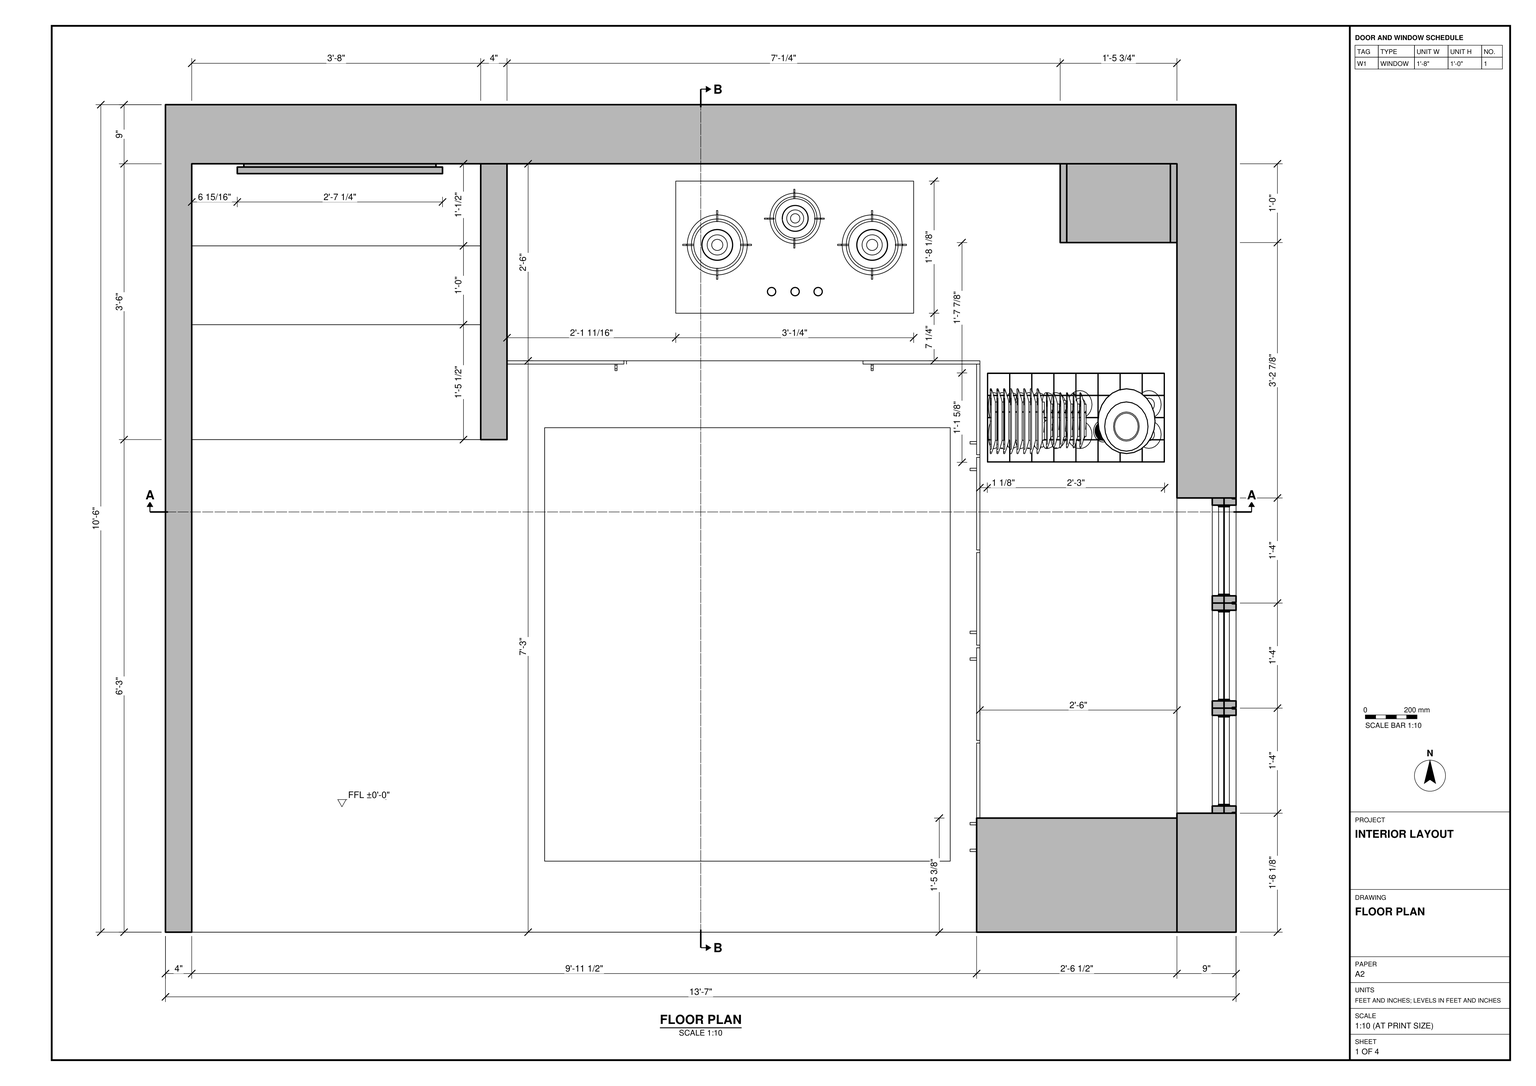
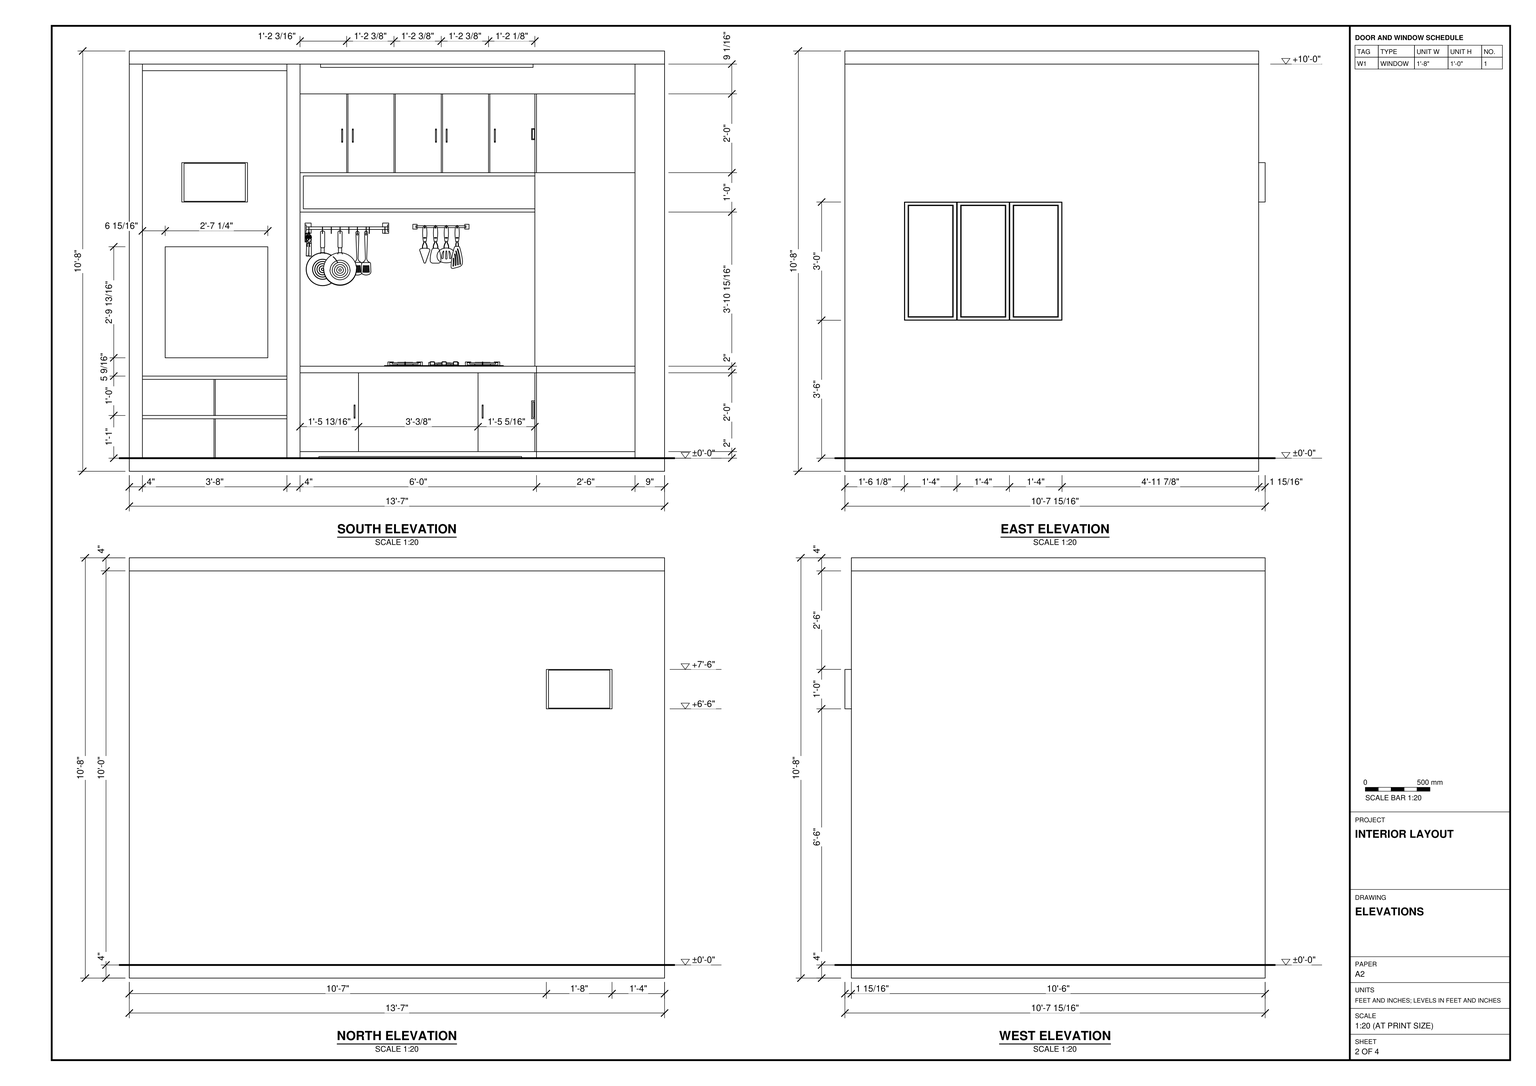
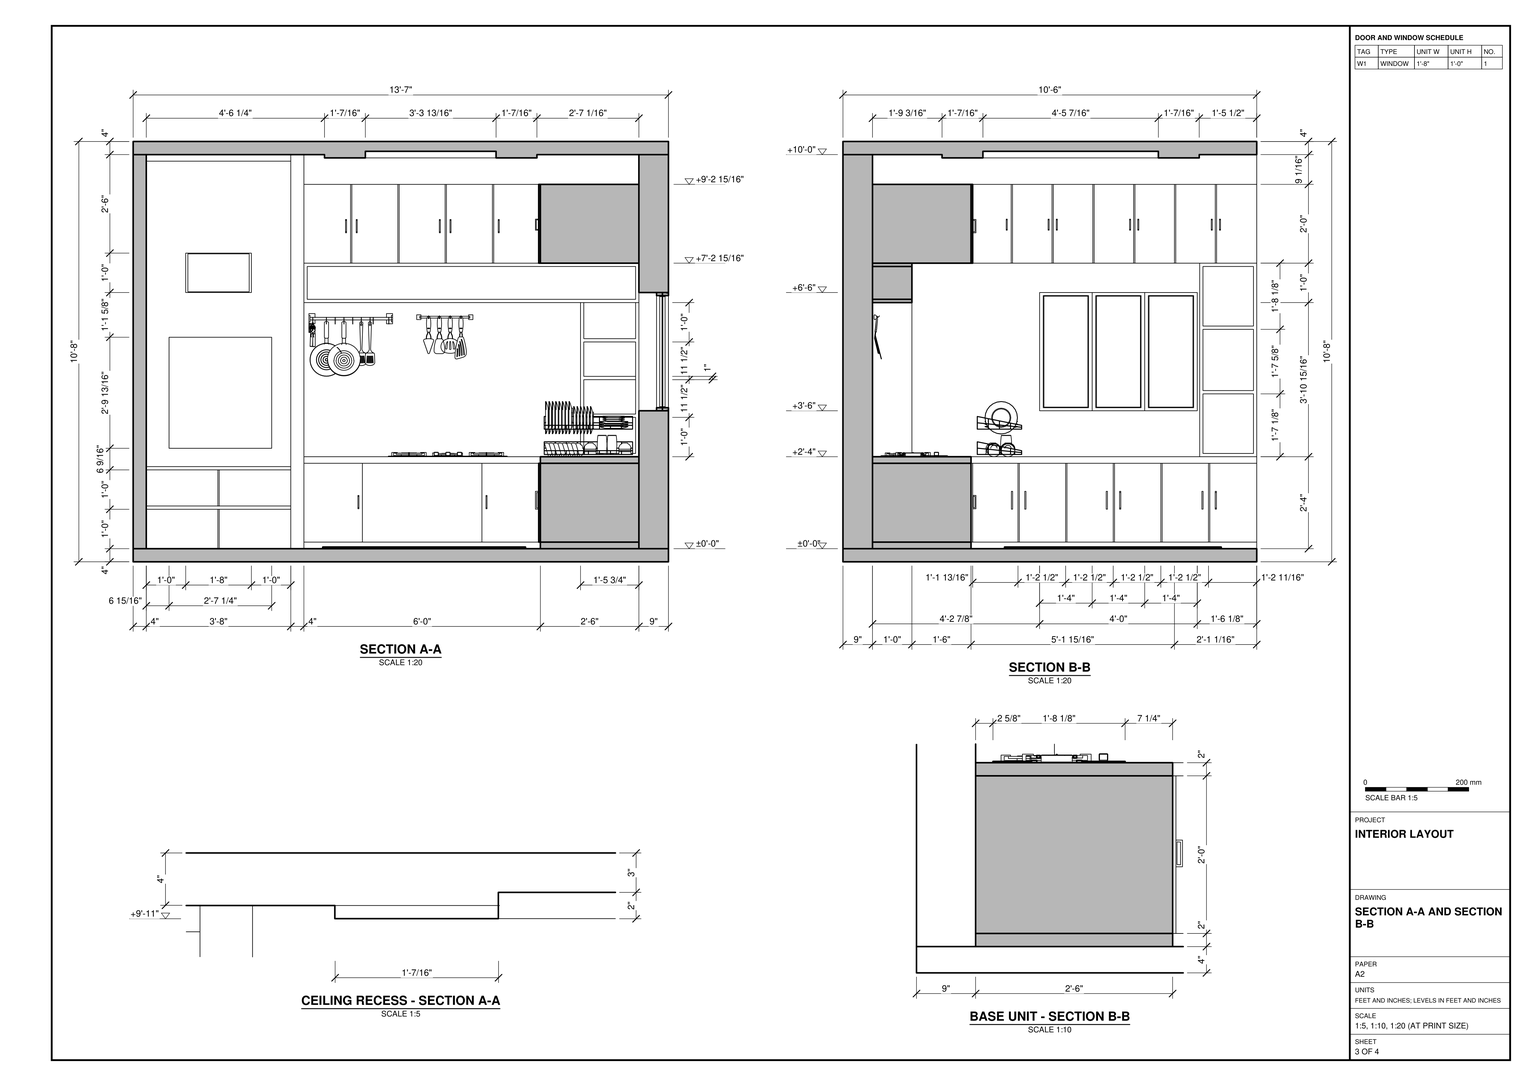
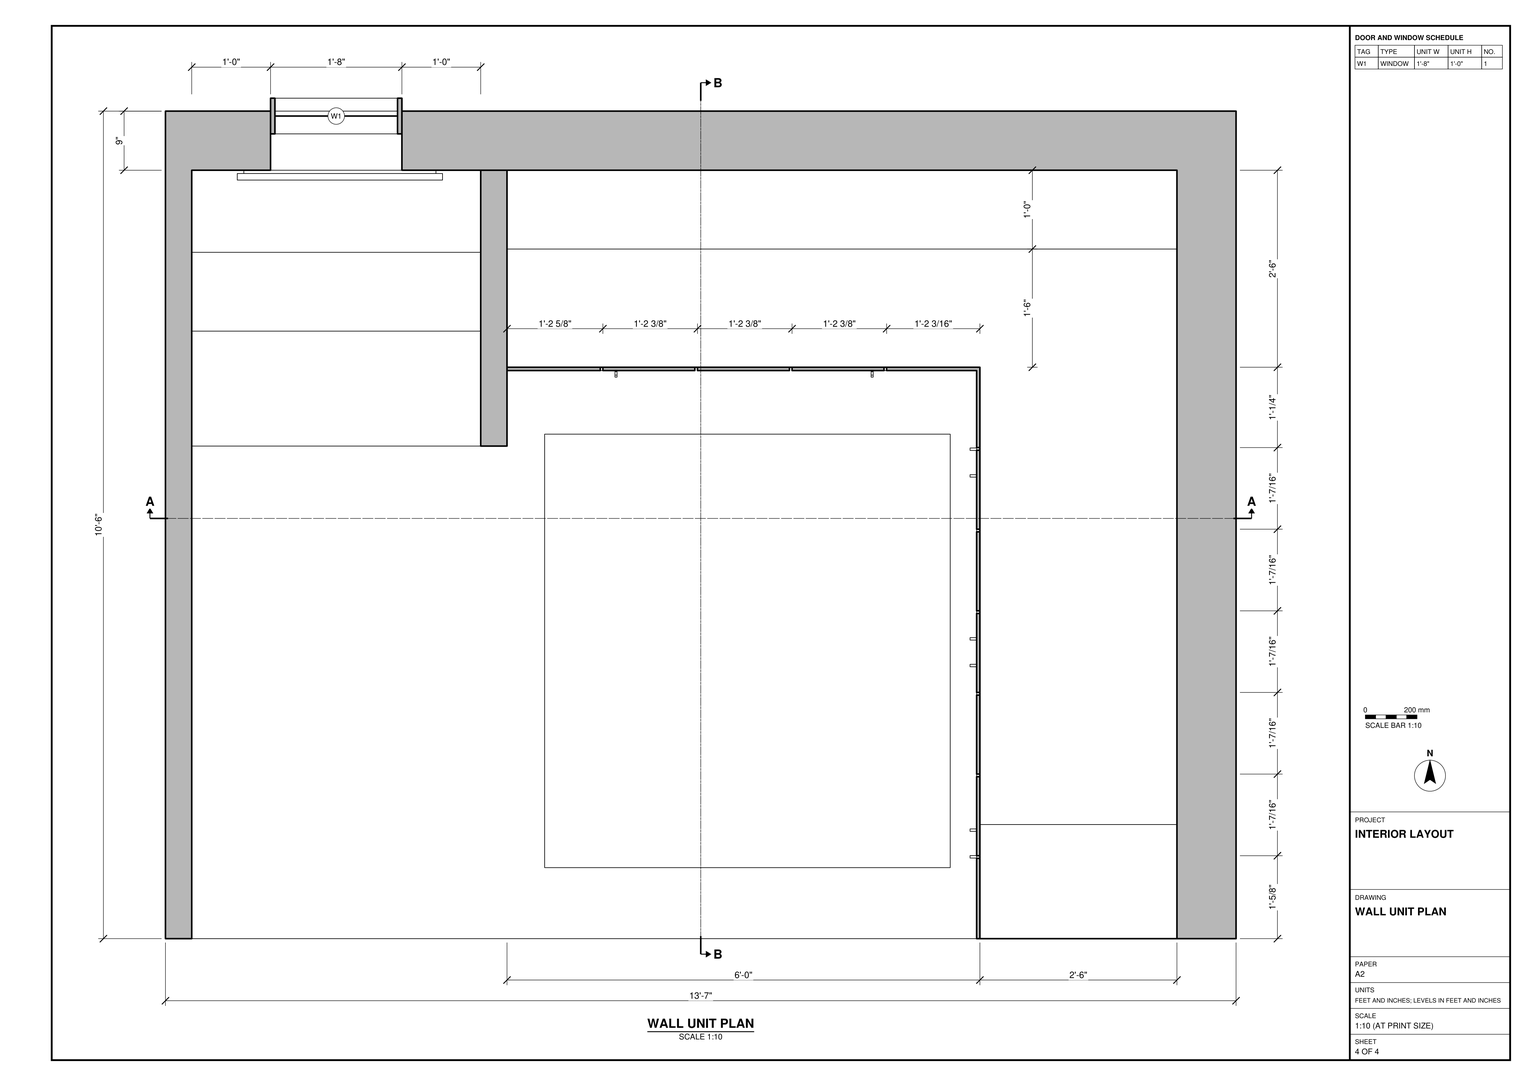
Build the kitchen interior in SketchUp from task_files/diagram_01.pdf. Work in feet and inches. The overall model extents are 13'-7" east to west, 10'-7 15/16" north to south and 10'-8" high. Set the single finished floor level at ±0'-0".

Use the floor plan for the wall positions and the sections for the floor slab, ceiling slab and ceiling recesses. Keep the south side open as drawn. Use 9" walls on the north and east, and 4" walls for the west side and the short partition beside the storage alcove. Model the small high window in the alcove and the three-panel glazed opening above the east counter.

Fit the base cabinets and continuous worktop along the north and east walls, leaving the centre of the room clear. Use the sections to set the counter height, cabinet fronts, plinths, pulls, upper cupboards and open shelves. Include the low divided shelving and wall panel in the alcove. Place the cooktop on the north counter, the hanging utensils above it and the dish rack near the corner on the east return. Decor and loose items may be any suitable library components, for example from 3D Warehouse.

Keep the shell elements and each joinery or furniture piece in separate groups or components, and use components for repeated parts. Save one SketchUp model as output_files/kitchen_with_l_shaped_cabinetry_and_storage_alcove.skp.

# SketchUp Ruby script. Lengths in inches.
U = 1.inch
M = Sketchup.active_model
def pt(a) = Geom::Point3d.new(a.map { |v| v * U })
def face(e, loops, mat)
  f = e.add_face(loops[0].map { |a| pt(a) })
  loops[1..].each { |l| e.add_face(l.map { |a| pt(a) }).erase! }
  f.material = f.back_material = mat if mat
  f
end
# faces: each face lists its corners as indices into pts; further lists are holes
def faces(e, pts, list, mat = nil) = list.each { |f| face(e, (f[0].is_a?(Array) ? f : [f]).map { |l| l.map { |i| pts[i] } }, mat) }
# xy, xz, yz: faces in a plane at the given z, y or x. An outline is a flat list of corners, or four numbers for a rectangle; further outlines are holes
def ring(l) = l.size == 4 ? [[l[0], l[1]], [l[2], l[1]], [l[2], l[3]], [l[0], l[3]]] : l.each_slice(2).to_a
def flat(e, list, mat, &to3) = list.each { |f| face(e, (f[0].is_a?(Array) ? f : [f]).map { |l| ring(l).map { |u, v| to3.(u, v) } }, mat) }
def xy(e, z, list, mat = nil) = flat(e, list, mat) { |x, y| [x, y, z] }
def xz(e, y, list, mat = nil) = flat(e, list, mat) { |x, z| [x, y, z] }
def yz(e, x, list, mat = nil) = flat(e, list, mat) { |y, z| [x, y, z] }
def lines(e, pts, list) = list.each { |a, b| e.add_line(pt(pts[a]), pt(pts[b])) }
# prism: a flat outline (further loops are holes) pulled along v
def prism(e, loops, v, mat = nil)
  f = face(e, loops, mat); d = Geom::Vector3d.new(v.map { |x| x * U })
  f.pushpull(f.normal.samedirection?(d) ? d.length : -d.length)
end
def box(e, o, s, mat = nil) = prism(e, [[o, [o[0] + s[0], o[1], o[2]], [o[0] + s[0], o[1] + s[1], o[2]], [o[0], o[1] + s[1], o[2]]]], [0, 0, s[2]], mat)
def at(x, y, z, deg = 0) = Geom::Transformation.translation(pt([x, y, z])) * Geom::Transformation.rotation(ORIGIN, Z_AXIS, deg.degrees)
def axes(o, x, y, z) = Geom::Transformation.new([*x, 0, *y, 0, *z, 0, *pt(o).to_a, 1])
def part(name) = M.definitions.add(name)
# library, detail: a bought-in or finely detailed component or shape, given as its bounding box
def library(name, o, s) = part(name).tap { |d| box(d.entities, o, s) }
def detail(e, o, s) = box(e.add_group.entities, o, s)
def put(e, d, t, mat = nil) = e.add_instance(d, t).tap { |i| i.material = mat if mat }
def group(e, t, mat = nil) = e.add_group.tap { |g| g.transformation = t; g.material = mat if mat }.entities
root = M.entities
M.materials.add("Emissive").color = [214, 204, 90]
M.materials.add("Wine2").color = [0, 0, 0]
M.materials["Wine2"].alpha = 0
M.materials.add("[0048_PaleGoldenrod]").color = [238, 232, 170]
M.materials.add("[0052_FloralWhite]").color = [255, 250, 240]
M.materials.add("[0055_LightGoldenrodYellow]").color = [250, 250, 210]
M.materials.add("[0057_DarkKhaki]").color = [189, 183, 107]
M.materials.add("[0130_Gainsboro]").color = [39, 45, 50]
M.materials.add("[Aluminum]").color = [179, 179, 179]
M.materials.add("[Carrera Marble]").color = [207, 207, 207]
M.materials.add("[Color M07]").color = [58, 58, 58]
M.materials.add("[Granite Dark Gray]").color = [69, 68, 68]
M.materials.add("[Stone Brushed Khaki]").color = [226, 197, 133]
M.materials.add("[Stone Vein Gray]").color = [166, 165, 165]
M.materials.add("[Textile Leaves Green]").color = [158, 160, 98]
M.materials.add("[Translucent Glass Gray]3").color = [128, 128, 128]
M.materials["[Translucent Glass Gray]3"].alpha = 0.3
M.materials.add("[Translucent Glass Sky Reflection]").color = [126, 138, 183]
M.materials["[Translucent Glass Sky Reflection]"].alpha = 0.52
c1 = part("Group14\#1")
p = [[0,0,0],[0,0,-15.5],[-7.68,0,-15.5],[50,-0.18,0],[-50,-0.18,0],[50,0.18,0],
  [50,0,0],[-50,0.18,0],[7.68,0,-15.5],[-50,0,0],[0,0,-25.09]]
lines(c1.entities,p,[[0,1],[1,2],[3,4],[5,6],[7,5],[1,8],[9,0],[0,6],[8,10],[4,9],[6,3],[2,10],
  [9,7]])
c2 = part("Rectangle Light")
put(c2.entities,c1,at(0,0,0))
c3 = part("WINDOW (1)")
xy(c3.entities,0,[[0,0,59.06,1.97]],"[Color M07]")
xy(c3.entities,1.97,[[1.97,0,57.09,0.98],[1.97,0.98,57.09,1.97]],"[Color M07]")
xy(c3.entities,104.33,[[1.97,0,57.09,0.98],[1.97,0.98,57.09,1.97]],"[Color M07]")
xy(c3.entities,106.3,[[0,0,59.06,1.97]],"[Color M07]")
xz(c3.entities,0,[[[0,0,59.06,106.3],[1.97,1.97,57.09,104.33]]],"[Color M07]")
xz(c3.entities,0.98,[[1.97,1.97,57.09,104.33]],"[Translucent Glass Gray]3")
xz(c3.entities,1.97,[[[0,0,59.06,106.3],[1.97,1.97,57.09,104.33]]],"[Color M07]")
yz(c3.entities,0,[[0,0,1.97,106.3]],"[Color M07]")
yz(c3.entities,1.97,[[0,1.97,0.98,104.33],[0.98,1.97,1.97,104.33]],"[Color M07]")
yz(c3.entities,57.09,[[0,1.97,0.98,104.33],[0.98,1.97,1.97,104.33]],"[Color M07]")
yz(c3.entities,59.06,[[0,0,1.97,106.3]],"[Color M07]")
c4 = part("Framed panel")
xy(c4.entities,0,[[0,-0.98,43.07,0],[0,0,43.07,1.4]],"[0130_Gainsboro]")
xy(c4.entities,0.3,[[0.3,-1.43,42.77,-0.98]],"[0130_Gainsboro]")
xy(c4.entities,2.95,[[2.95,-1.43,40.12,-0.63],[2.95,-0.63,40.12,0],[2.95,0,40.12,0.64],[2.95,0.64,40.12,1.4]],"[0130_Gainsboro]")
xy(c4.entities,3.54,[[3.54,-0.63,39.53,0],[3.54,0,39.53,0.64]],"[0130_Gainsboro]")
xy(c4.entities,111.8125,[[3.54,-0.63,39.53,0],[3.54,0,39.53,0.64]],"[0130_Gainsboro]")
xy(c4.entities,112.4,[[2.95,-1.43,40.12,-0.63],[2.95,-0.63,40.12,0],[2.95,0,40.12,0.64],[2.95,0.64,40.12,1.4]],"[0130_Gainsboro]")
xy(c4.entities,115.05,[[0.3,-1.43,42.77,-0.98]],"[0130_Gainsboro]")
xy(c4.entities,115.35,[[0,-0.98,43.07,0],[0,0,43.07,1.4]],"[0130_Gainsboro]")
xz(c4.entities,-1.43,[[[0.3,0.3,42.77,115.05],[2.95,2.95,40.12,112.4]]],"[0130_Gainsboro]")
xz(c4.entities,-0.98,[[[0,0,43.07,115.35],[0.3,0.3,42.77,115.05]]],"[0130_Gainsboro]")
xz(c4.entities,-0.63,[[[2.95,2.95,40.12,112.4],[3.54,3.54,39.53,111.8125]]],"[0130_Gainsboro]")
xz(c4.entities,0,[[3.54,3.54,39.53,111.8125]],"Wine2")
xz(c4.entities,0,[[[0,0,43.07,115.35],[2.95,2.95,40.12,112.4]],[[2.95,2.95,40.12,112.4],[3.54,3.54,39.53,111.8125]]],"[0130_Gainsboro]")
xz(c4.entities,0.64,[[[2.95,2.95,40.12,112.4],[3.54,3.54,39.53,111.8125]]],"[0130_Gainsboro]")
xz(c4.entities,1.4,[[[0,0,43.07,115.35],[2.95,2.95,40.12,112.4]]],"[0130_Gainsboro]")
yz(c4.entities,0,[[-0.98,0,0,115.35],[0,0,1.4,115.35]],"[0130_Gainsboro]")
yz(c4.entities,0.3,[[-1.43,0.3,-0.98,115.05]],"[0130_Gainsboro]")
yz(c4.entities,2.95,[[-1.43,2.95,-0.63,112.4],[-0.63,2.95,0,112.4],[0,2.95,0.64,112.4],[0.64,2.95,1.4,112.4]],"[0130_Gainsboro]")
yz(c4.entities,3.54,[[-0.63,3.54,0,111.8125],[0,3.54,0.64,111.8125]],"[0130_Gainsboro]")
yz(c4.entities,39.53,[[-0.63,3.54,0,111.8125],[0,3.54,0.64,111.8125]],"[0130_Gainsboro]")
yz(c4.entities,40.12,[[-1.43,2.95,-0.63,112.4],[-0.63,2.95,0,112.4],[0,2.95,0.64,112.4],[0.64,2.95,1.4,112.4]],"[0130_Gainsboro]")
yz(c4.entities,42.77,[[-1.43,0.3,-0.98,115.05]],"[0130_Gainsboro]")
yz(c4.entities,43.07,[[-0.98,0,0,115.35],[0,0,1.4,115.35]],"[0130_Gainsboro]")
c5 = part("Framed panel assembly")
put(c5.entities,c4,axes([90.57,1.43,0],[1.05148,0,0],[0,1,0],[0,0,1]))
put(c5.entities,c4,axes([0,1.43,0],[1.05148,0,0],[0,1,0],[0,0,1]))
put(c5.entities,c4,axes([45.29,1.43,0],[1.05148,0,0],[0,1,0],[0,0,1]))
c6 = library("Bosch Stove",[0,0,0],[36.22,20.12,1.38])
c7 = library("FF_Model_ID4182_2_FrypancoatedCF2SU5",[11.81,0,-0.01],[31.3,13.89,17.18])
c8 = library("kitchen+utensils",[-0.01,-12.39,-0.45],[15.99,12.58,3.71])
c9 = library("Cookware hanging rack",[-2.09,-19.1875,0],[25.71,19.1875,6.07])
c10 = part("Group\#7")
prism(c10.entities,[[[72,87,0],[0,87,0],[0,117,0],[102,117,0],[102,0,0],[72,0,0]]],[0,0,2])
c11 = part("Group\#14")
prism(c11.entities,[[[0,1,4.0625],[0,1,0],[0,0,0],[0,0,4.0625]],[[0,0.3,0.3],[0,0.83,0.34],[0,0.83,3.8],[0,0.3,3.76]]],[0.3125,0,0])
c12 = part("Group\#16")
prism(c12.entities,[[[1,0.375,5.4375],[1,0.375,0],[0,0.375,0],[0,0.375,5.4375]],[[0.77,0.375,0.35],[0.77,0.375,5.08],[0.35,0.375,5.08],[0.35,0.375,0.35]]],[0,-0.375,0])
c13 = part("Group\#17")
prism(c13.entities,[[[1,0,0],[1,0,3.375],[0,0,3.375],[0,0,0]],[[0.88,0,3.13],[0.88,0,0.24],[0.24,0,0.24],[0.24,0,3.13]]],[0,0.3125,0])
xy(root,4,[[57.73,10.8125,119.48,76.8125],[4,92.5,25.8,93],[26.2,92.5,48,93]])
xy(root,4.5,[[57.73,10.8125,119.48,76.8125]],"[Textile Leaves Green]")
xy(root,16,[[25.8,92.5,25.8,93,4,93,4,104.5,25.8,104.5,25.8,105,26.2,105,26.2,104.5,48,104.5,48,93,26.2,93,26.2,92.5],[4,92.5,25.8,93],[26.2,92.5,48,93],[4,104.5,25.8,105],[26.2,104.5,48,105]])
xy(root,17,[[4,92.5,48,92.5,48,104.5,26.2,104.5,26.2,105,25.8,105,25.8,104.5,4,104.5]],"[Carrera Marble]")
xy(root,28,[[25.8,104.5,25.8,105,4,105,4,117,48,117,48,105,26.2,105,26.2,104.5],[4,104.5,25.8,105],[26.2,104.5,48,105]])
xy(root,29,[[4,104.5,48,117]],"[Carrera Marble]")
xy(root,34.57,[[10.93,115.5,42.18,116.5]])
xy(root,68.38,[[10.93,115.5,42.18,116.5]])
xy(root,122,[[[4,75,48,117],[24.76,77.75,25.14,77.75,25.52,77.76,25.91,77.78,26.29,77.8125,26.67,77.85,27.05,77.9,27.43,77.96,27.8,78.03,28.18,78.11,28.92,78.29,29.29,78.4,29.65,78.52,30.37,78.78,30.73,78.93,31.08,79.08,31.76,79.42,32.1,79.6,32.43,79.79,32.76,79.99,33.08,80.2,33.4,80.42,33.71,80.64,34.31,81.11,34.6,81.36,35.16,81.88,35.43,82.15,35.7,82.43,35.96,82.71,36.2,83,36.45,83.3,36.68,83.6,36.91,83.91,37.33,84.55,37.53,84.875,37.73,85.21,37.91,85.54,38.08,85.88,38.25,86.23,38.55,86.93,38.69,87.29,38.82,87.65,38.9375,88.01,39.05,88.38,39.15,88.75,39.24,89.12,39.32,89.5,39.39,89.87,39.45,90.25,39.5,90.63,39.54,91.01,39.57,91.39,39.59,91.77,39.6,92.16,39.6,92.54,39.59,92.92,39.57,93.3,39.55,93.6875,39.51,94.07,39.46,94.45,39.4,94.83,39.33,95.2,39.25,95.58,39.16,95.95,39.0625,96.32,38.96,96.6875,38.84,97.05,38.71,97.41,38.57,97.77,38.43,98.125,38.27,98.47,38.11,98.82,37.9375,99.16,37.75,99.5,37.5625,99.83,37.36,100.16,37.16,100.48,36.72,101.1,36.48,101.41,36.24,101.71,35.99,102,35.74,102.28,35.48,102.5625,35.21,102.83,34.93,103.1,34.35,103.6,34.06,103.84,33.75,104.08,33.13,104.52,32.81,104.73,32.48,104.93,32.15,105.125,31.82,105.31,31.47,105.48,31.13,105.65,30.43,105.95,30.07,106.09,29.71,106.22,29.34,106.34,28.98,106.45,28.61,106.55,28.24,106.64,27.86,106.72,27.49,106.79,27.11,106.85,26.73,106.9,26.35,106.9375,25.97,106.97,25.58,106.99,25.2,107,24.82,107,24.43,106.99,24.05,106.97,23.29,106.91,22.91,106.86,22.53,106.8,22.16,106.73,21.78,106.65,21.41,106.56,21.04,106.46,20.67,106.35,20.31,106.24,19.95,106.11,19.23,105.83,18.88,105.67,18.54,105.51,17.86,105.15,17.53,104.96,17.2,104.76,16.88,104.55,16.5625,104.34,16.25,104.11,15.95,103.88,15.65,103.64,15.07,103.14,14.8,102.875,14.52,102.6,14.26,102.33,14,102.04,13.75,101.75,13.51,101.46,13.05,100.84,12.84,100.53,12.625,100.21,12.43,99.88,12.23,99.55,12.05,99.21,11.875,98.875,11.71,98.53,11.55,98.18,11.41,97.82,11.27,97.47,11.14,97.11,11.02,96.74,10.91,96.375,10.8125,96.01,10.72,95.63,10.64,95.26,10.57,94.88,10.51,94.51,10.46,94.125,10.42,93.75,10.39,93.36,10.37,92.98,10.36,92.6,10.36,91.83,10.38,91.45,10.41,91.07,10.45,90.6875,10.5,90.31,10.5625,89.93,10.63,89.55,10.71,89.18,10.8,88.81,10.9,88.4375,11,88.07,11.12,87.71,11.25,87.34,11.38,86.99,11.53,86.63,11.69,86.28,11.85,85.9375,12.02,85.59,12.2,85.26,12.4,84.93,12.59,84.6,12.8,84.28,13.02,83.96,13.24,83.65,13.72,83.05,13.96,82.76,14.22,82.47,14.48,82.19,14.75,81.92,15.03,81.66,15.3125,81.4,15.6,81.15,15.9,80.91,16.2,80.68,16.51,80.45,16.83,80.23,17.15,80.03,17.48,79.82,17.81,79.63,18.14,79.45,18.48,79.27,19.18,78.95,19.53,78.81,19.89,78.67,20.25,78.54,20.61,78.42,20.98,78.31,21.35,78.21,21.72,78.12,22.1,78.04,22.47,77.97,22.85,77.91,23.23,77.86,23.61,77.82,23.99,77.79]]])
xy(root,123,[[[58.27,17.51,122.95,95.83],[70.71,29.96,110.51,83.38]],[24.76,77.75,23.99,77.79,23.61,77.82,23.23,77.86,22.85,77.91,22.47,77.97,22.1,78.04,21.72,78.12,21.35,78.21,20.98,78.31,20.61,78.42,20.25,78.54,19.89,78.67,19.53,78.81,19.18,78.95,18.48,79.27,18.14,79.45,17.81,79.63,17.48,79.82,17.15,80.03,16.83,80.23,16.51,80.45,16.2,80.68,15.9,80.91,15.6,81.15,15.3125,81.4,15.03,81.66,14.75,81.92,14.48,82.19,14.22,82.47,13.96,82.76,13.72,83.05,13.24,83.65,13.02,83.96,12.8,84.28,12.59,84.6,12.4,84.93,12.2,85.26,12.02,85.59,11.85,85.9375,11.69,86.28,11.53,86.63,11.38,86.99,11.25,87.34,11.12,87.71,11,88.07,10.9,88.4375,10.8,88.81,10.71,89.18,10.63,89.55,10.5625,89.93,10.5,90.31,10.45,90.6875,10.41,91.07,10.38,91.45,10.36,91.83,10.36,92.6,10.37,92.98,10.39,93.36,10.42,93.75,10.46,94.125,10.51,94.51,10.57,94.88,10.64,95.26,10.72,95.63,10.8125,96.01,10.91,96.375,11.02,96.74,11.14,97.11,11.27,97.47,11.41,97.82,11.55,98.18,11.71,98.53,11.875,98.875,12.05,99.21,12.23,99.55,12.43,99.88,12.625,100.21,12.84,100.53,13.05,100.84,13.51,101.46,13.75,101.75,14,102.04,14.26,102.33,14.52,102.6,14.8,102.875,15.07,103.14,15.65,103.64,15.95,103.88,16.25,104.11,16.5625,104.34,16.88,104.55,17.2,104.76,17.53,104.96,17.86,105.15,18.54,105.51,18.88,105.67,19.23,105.83,19.95,106.11,20.31,106.24,20.67,106.35,21.04,106.46,21.41,106.56,21.78,106.65,22.16,106.73,22.53,106.8,22.91,106.86,23.29,106.91,24.05,106.97,24.43,106.99,24.82,107,25.2,107,25.58,106.99,25.97,106.97,26.35,106.9375,26.73,106.9,27.11,106.85,27.49,106.79,27.86,106.72,28.24,106.64,28.61,106.55,28.98,106.45,29.34,106.34,29.71,106.22,30.07,106.09,30.43,105.95,31.13,105.65,31.47,105.48,31.82,105.31,32.15,105.125,32.48,104.93,32.81,104.73,33.13,104.52,33.75,104.08,34.06,103.84,34.35,103.6,34.93,103.1,35.21,102.83,35.48,102.5625,35.74,102.28,35.99,102,36.24,101.71,36.48,101.41,36.72,101.1,37.16,100.48,37.36,100.16,37.5625,99.83,37.75,99.5,37.9375,99.16,38.11,98.82,38.27,98.47,38.43,98.125,38.57,97.77,38.71,97.41,38.84,97.05,38.96,96.6875,39.0625,96.32,39.16,95.95,39.25,95.58,39.33,95.2,39.4,94.83,39.46,94.45,39.51,94.07,39.55,93.6875,39.57,93.3,39.59,92.92,39.6,92.54,39.6,92.16,39.59,91.77,39.57,91.39,39.54,91.01,39.5,90.63,39.45,90.25,39.39,89.87,39.32,89.5,39.24,89.12,39.15,88.75,39.05,88.38,38.9375,88.01,38.82,87.65,38.69,87.29,38.55,86.93,38.25,86.23,38.08,85.88,37.91,85.54,37.73,85.21,37.53,84.875,37.33,84.55,36.91,83.91,36.68,83.6,36.45,83.3,36.2,83,35.96,82.71,35.7,82.43,35.43,82.15,35.16,81.88,34.6,81.36,34.31,81.11,33.71,80.64,33.4,80.42,33.08,80.2,32.76,79.99,32.43,79.79,32.1,79.6,31.76,79.42,31.08,79.08,30.73,78.93,30.37,78.78,29.65,78.52,29.29,78.4,28.92,78.29,28.18,78.11,27.8,78.03,27.43,77.96,27.05,77.9,26.67,77.85,26.29,77.8125,25.91,77.78,25.52,77.76,25.14,77.75]])
xy(root,124,[[[0,0,163,126],[58.27,17.51,122.95,95.83],[4,75,48,117]]])
xy(root,125,[[70.71,29.96,110.51,83.38]])
xy(root,128,[[0,0,163,126]])
xz(root,0,[[0,124,163,128]])
xz(root,10.8125,[[57.73,4,119.48,4.5]])
xz(root,17.51,[[58.27,123,122.95,124]])
xz(root,29.96,[[70.71,123,110.51,125]],"Emissive")
xz(root,75,[[4,122,48,124]])
xz(root,76.8125,[[57.73,4,119.48,4.5]])
xz(root,77.75,[[24.76,122,25.14,123]],"Emissive")
xz(root,83.38,[[70.71,123,110.51,125]],"Emissive")
xz(root,92.5,[[4,4,25.8,16]])
xz(root,92.5,[[26.2,4,48,16]],"[0055_LightGoldenrodYellow]")
xz(root,92.5,[[4,16,48,17]],"[Carrera Marble]")
xz(root,93,[[4,4,25.8,16],[26.2,4,48,16]])
xz(root,95.83,[[58.27,123,122.95,124]])
xz(root,104.5,[[4,16,25.8,17],[26.2,16,48,17],[4,17,25.8,28]])
xz(root,104.5,[[26.2,17,48,28]],"[0055_LightGoldenrodYellow]")
xz(root,104.5,[[4,28,48,29]],"[Carrera Marble]")
xz(root,105,[[4,16,25.8,28],[25.8,16,26.2,17],[26.2,16,48,28]])
xz(root,105,[[137.22,33,153,43.98],[137.22,44.98,153,55.47],[137.22,56.47,153,66.95],[137.22,67.95,153,78.9375],[53,79.9375,153,89.9375]],"[Translucent Glass Sky Reflection]")
xz(root,107,[[24.82,122,25.2,123]],"Emissive")
xz(root,115.5,[[10.93,34.57,42.18,68.38]],"[Stone Brushed Khaki]")
xz(root,116.5,[[10.93,34.57,42.18,68.38]])
xz(root,117,[[4,28,48,29],[4,122,48,124]])
xz(root,117,[[137.22,42.79,153,43.98],[137.22,54.4375,153,55.47],[137.22,66.16,153,66.95],[137.22,78.05,153,78.9375]],"Emissive")
xz(root,126,[[0,124,163,128]])
yz(root,0,[[0,124,126,128]])
yz(root,4,[[92.5,4,93,16],[92.5,16,104.5,17],[104.5,16,105,28],[104.5,28,117,29],[75,122,117,124]])
yz(root,10.36,[[91.83,122,92.22,123],[92.22,122,92.6,123]],"Emissive")
yz(root,10.93,[[115.5,34.57,116.5,68.38]])
yz(root,25.8,[[92.5,4,93,16],[104.5,16,105,17],[104.5,17,105,28]])
yz(root,26.2,[[92.5,4,93,16],[104.5,16,105,17],[104.5,17,105,28]])
yz(root,39.6,[[92.16,122,92.54,123]],"Emissive")
yz(root,42.18,[[115.5,34.57,116.5,68.38]])
yz(root,48,[[92.5,4,93,16],[92.5,16,104.5,17],[104.5,16,105,28],[104.5,28,117,29],[75,122,117,124]])
yz(root,57.73,[[10.8125,4,76.8125,4.5]])
yz(root,58.27,[[17.51,123,95.83,124]])
yz(root,70.71,[[29.96,123,83.38,125]],"Emissive")
yz(root,110.51,[[29.96,123,83.38,125]],"Emissive")
yz(root,119.48,[[10.8125,4,76.8125,4.5]])
yz(root,122.95,[[17.51,123,95.83,124]])
yz(root,123.5,[[1,33,16.375,51.15],[1,52.15,16.375,70.79],[1,71.79,16.375,89.9375]],"[Translucent Glass Sky Reflection]")
yz(root,154,[[1,49.6,16.375,51.15],[1,69.55,16.375,70.79],[1,88.93,16.375,89.9375]],"Emissive")
yz(root,163,[[0,124,126,128]])
p = [[23.61,77.82,122],[23.23,77.86,122],[23.23,77.86,123],[23.61,77.82,123],[23.99,77.79,122],[23.99,77.79,123],
  [24.375,77.77,122],[24.375,77.77,123],[24.76,77.75,122],[24.76,77.75,123],[25.52,77.76,122],[25.14,77.75,122],
  [25.14,77.75,123],[25.52,77.76,123],[25.91,77.78,122],[25.91,77.78,123],[26.29,77.8125,122],[26.29,77.8125,123],
  [26.67,77.85,122],[26.67,77.85,123],[22.85,77.91,122],[22.47,77.97,122],[22.47,77.97,123],[22.85,77.91,123],
  [27.05,77.9,122],[27.05,77.9,123],[27.43,77.96,122],[27.43,77.96,123],[22.1,78.04,122],[21.72,78.12,122],
  [21.72,78.12,123],[22.1,78.04,123],[27.8,78.03,122],[27.8,78.03,123],[28.18,78.11,122],[28.18,78.11,123],
  [21.35,78.21,122],[21.35,78.21,123],[28.55,78.2,122],[28.55,78.2,123],[20.98,78.31,122],[20.98,78.31,123],
  [28.92,78.29,122],[28.92,78.29,123],[20.61,78.42,122],[20.61,78.42,123],[29.29,78.4,122],[29.29,78.4,123],
  [20.25,78.54,122],[20.25,78.54,123],[29.65,78.52,122],[29.65,78.52,123],[19.89,78.67,122],[19.89,78.67,123],
  [30.01,78.65,122],[30.01,78.65,123],[30.37,78.78,122],[30.37,78.78,123],[19.53,78.81,122],[19.53,78.81,123],
  [19.18,78.95,122],[19.18,78.95,123],[30.73,78.93,122],[30.73,78.93,123],[31.08,79.08,122],[31.08,79.08,123],
  [18.83,79.11,122],[18.83,79.11,123],[18.48,79.27,122],[18.48,79.27,123],[31.42,79.25,122],[31.42,79.25,123],
  [31.76,79.42,122],[31.76,79.42,123],[18.14,79.45,122],[18.14,79.45,123],[17.81,79.63,122],[17.81,79.63,123],
  [32.1,79.6,122],[32.1,79.6,123],[17.48,79.82,122],[17.48,79.82,123],[32.43,79.79,122],[32.43,79.79,123],
  [17.15,80.03,122],[17.15,80.03,123],[32.76,79.99,122],[32.76,79.99,123],[16.83,80.23,122],[16.83,80.23,123],
  [33.08,80.2,122],[33.08,80.2,123],[16.51,80.45,122],[16.51,80.45,123],[33.4,80.42,122],[33.4,80.42,123],
  [33.71,80.64,122],[33.71,80.64,123],[16.2,80.68,122],[16.2,80.68,123],[34.01,80.875,122],[34.01,80.875,123],
  [15.9,80.91,122],[15.9,80.91,123],[15.6,81.15,122],[15.6,81.15,123],[34.31,81.11,122],[34.31,81.11,123],
  [34.6,81.36,122],[34.6,81.36,123],[15.3125,81.4,122],[15.3125,81.4,123],[15.03,81.66,122],[15.03,81.66,123],
  [34.88,81.62,122],[34.88,81.62,123],[35.16,81.88,122],[35.16,81.88,123],[14.75,81.92,122],[14.75,81.92,123],
  [14.48,82.19,122],[14.48,82.19,123],[35.43,82.15,122],[35.43,82.15,123],[14.22,82.47,122],[14.22,82.47,123],
  [35.7,82.43,122],[35.7,82.43,123],[35.96,82.71,122],[35.96,82.71,123],[13.96,82.76,122],[13.96,82.76,123],
  [36.2,83,122],[36.2,83,123],[13.72,83.05,122],[13.72,83.05,123],[13.48,83.35,122],[13.48,83.35,123],
  [36.45,83.3,122],[36.45,83.3,123],[13.24,83.65,122],[13.24,83.65,123],[36.68,83.6,122],[36.68,83.6,123],
  [36.91,83.91,122],[36.91,83.91,123],[13.02,83.96,122],[13.02,83.96,123],[37.12,84.23,122],[37.12,84.23,123],
  [12.8,84.28,122],[12.8,84.28,123],[37.33,84.55,122],[37.33,84.55,123],[12.59,84.6,122],[12.59,84.6,123],
  [37.53,84.875,122],[37.53,84.875,123],[12.4,84.93,122],[12.4,84.93,123],[12.2,85.26,122],[12.2,85.26,123],
  [37.73,85.21,122],[37.73,85.21,123],[37.91,85.54,122],[37.91,85.54,123],[12.02,85.59,122],[12.02,85.59,123],
  [38.08,85.88,122],[38.08,85.88,123],[11.85,85.9375,122],[11.85,85.9375,123],[11.69,86.28,122],[11.69,86.28,123],
  [38.25,86.23,122],[38.25,86.23,123],[38.4,86.58,122],[38.4,86.58,123],[11.53,86.63,122],[11.53,86.63,123],
  [11.38,86.99,122],[11.38,86.99,123],[38.55,86.93,122],[38.55,86.93,123],[38.69,87.29,122],[38.69,87.29,123],
  [11.25,87.34,122],[11.25,87.34,123],[11.12,87.71,122],[11.12,87.71,123],[38.82,87.65,122],[38.82,87.65,123],
  [38.9375,88.01,122],[38.9375,88.01,123],[11,88.07,122],[11,88.07,123],[39.05,88.38,122],[39.05,88.38,123],
  [10.9,88.4375,122],[10.9,88.4375,123],[10.8,88.81,122],[10.8,88.81,123],[39.15,88.75,122],[39.15,88.75,123],
  [39.24,89.12,122],[39.24,89.12,123],[10.71,89.18,122],[10.71,89.18,123],[39.32,89.5,122],[39.32,89.5,123],
  [10.63,89.55,122],[10.63,89.55,123],[39.39,89.87,122],[39.39,89.87,123],[10.5625,89.93,122],[10.5625,89.93,123],
  [10.5,90.31,122],[10.5,90.31,123],[39.45,90.25,122],[39.45,90.25,123],[39.5,90.63,122],[39.5,90.63,123],
  [10.45,90.6875,122],[10.45,90.6875,123],[39.54,91.01,122],[39.54,91.01,123],[10.41,91.07,122],[10.41,91.07,123],
  [39.57,91.39,122],[39.57,91.39,123],[10.38,91.45,122],[10.38,91.45,123],[39.59,91.77,122],[39.59,91.77,123],
  [10.36,91.83,122],[10.36,91.83,123],[39.6,92.16,122],[39.6,92.16,123],[39.59,92.92,122],[39.6,92.54,122],
  [39.6,92.54,123],[39.59,92.92,123],[10.36,92.6,122],[10.37,92.98,122],[10.37,92.98,123],[10.36,92.6,123],
  [39.57,93.3,122],[39.57,93.3,123],[10.39,93.36,122],[10.39,93.36,123],[39.55,93.6875,122],[39.55,93.6875,123],
  [10.42,93.75,122],[10.42,93.75,123],[10.46,94.125,122],[10.46,94.125,123],[39.51,94.07,122],[39.51,94.07,123],
  [10.51,94.51,122],[10.51,94.51,123],[39.46,94.45,122],[39.46,94.45,123],[39.4,94.83,122],[39.4,94.83,123],
  [10.57,94.88,122],[10.57,94.88,123],[39.33,95.2,122],[39.33,95.2,123],[10.64,95.26,122],[10.64,95.26,123],
  [39.25,95.58,122],[39.25,95.58,123],[10.72,95.63,122],[10.72,95.63,123],[10.8125,96.01,122],[10.8125,96.01,123],
  [39.16,95.95,122],[39.16,95.95,123],[39.0625,96.32,122],[39.0625,96.32,123],[10.91,96.375,122],[10.91,96.375,123],
  [38.96,96.6875,122],[38.96,96.6875,123],[11.02,96.74,122],[11.02,96.74,123],[11.14,97.11,122],[11.14,97.11,123],
  [38.84,97.05,122],[38.84,97.05,123],[11.27,97.47,122],[11.27,97.47,123],[38.71,97.41,122],[38.71,97.41,123],
  [38.57,97.77,122],[38.57,97.77,123],[11.41,97.82,122],[11.41,97.82,123],[11.55,98.18,122],[11.55,98.18,123],
  [38.43,98.125,122],[38.43,98.125,123],[38.27,98.47,122],[38.27,98.47,123],[11.71,98.53,122],[11.71,98.53,123],
  [11.875,98.875,122],[11.875,98.875,123],[38.11,98.82,122],[38.11,98.82,123],[37.9375,99.16,122],[37.9375,99.16,123],
  [12.05,99.21,122],[12.05,99.21,123],[12.23,99.55,122],[12.23,99.55,123],[37.75,99.5,122],[37.75,99.5,123],
  [12.43,99.88,122],[12.43,99.88,123],[37.5625,99.83,122],[37.5625,99.83,123],[37.36,100.16,122],[37.36,100.16,123],
  [12.625,100.21,122],[12.625,100.21,123],[12.84,100.53,122],[12.84,100.53,123],[37.16,100.48,122],[37.16,100.48,123],
  [13.05,100.84,122],[13.05,100.84,123],[36.94,100.79,122],[36.94,100.79,123],[13.28,101.15,122],[13.28,101.15,123],
  [36.72,101.1,122],[36.72,101.1,123],[36.48,101.41,122],[36.48,101.41,123],[13.51,101.46,122],[13.51,101.46,123],
  [36.24,101.71,122],[36.24,101.71,123],[13.75,101.75,122],[13.75,101.75,123],[35.99,102,122],[35.99,102,123],
  [14,102.04,122],[14,102.04,123],[14.26,102.33,122],[14.26,102.33,123],[35.74,102.28,122],[35.74,102.28,123],
  [14.52,102.6,122],[14.52,102.6,123],[35.48,102.5625,122],[35.48,102.5625,123],[14.8,102.875,122],[14.8,102.875,123],
  [35.21,102.83,122],[35.21,102.83,123],[34.93,103.1,122],[34.93,103.1,123],[15.07,103.14,122],[15.07,103.14,123],
  [15.36,103.39,122],[15.36,103.39,123],[34.64,103.35,122],[34.64,103.35,123],[15.65,103.64,122],[15.65,103.64,123],
  [34.35,103.6,122],[34.35,103.6,123],[15.95,103.88,122],[15.95,103.88,123],[34.06,103.84,122],[34.06,103.84,123],
  [33.75,104.08,122],[33.75,104.08,123],[16.25,104.11,122],[16.25,104.11,123],[16.5625,104.34,122],[16.5625,104.34,123],
  [33.44,104.3,122],[33.44,104.3,123],[16.88,104.55,122],[16.88,104.55,123],[33.13,104.52,122],[33.13,104.52,123],
  [32.81,104.73,122],[32.81,104.73,123],[17.2,104.76,122],[17.2,104.76,123],[32.48,104.93,122],[32.48,104.93,123],
  [17.53,104.96,122],[17.53,104.96,123],[32.15,105.125,122],[32.15,105.125,123],[17.86,105.15,122],[17.86,105.15,123],
  [31.82,105.31,122],[31.82,105.31,123],[18.2,105.33,122],[18.2,105.33,123],[18.54,105.51,122],[18.54,105.51,123],
  [31.47,105.48,122],[31.47,105.48,123],[18.88,105.67,122],[18.88,105.67,123],[31.13,105.65,122],[31.13,105.65,123],
  [30.78,105.8,122],[30.78,105.8,123],[19.23,105.83,122],[19.23,105.83,123],[19.59,105.97,122],[19.59,105.97,123],
  [30.43,105.95,122],[30.43,105.95,123],[19.95,106.11,122],[19.95,106.11,123],[30.07,106.09,122],[30.07,106.09,123],
  [20.31,106.24,122],[20.31,106.24,123],[29.71,106.22,122],[29.71,106.22,123],[20.67,106.35,122],[20.67,106.35,123],
  [29.34,106.34,122],[29.34,106.34,123],[28.98,106.45,122],[28.98,106.45,123],[21.04,106.46,122],[21.04,106.46,123],
  [28.61,106.55,122],[28.61,106.55,123],[21.41,106.56,122],[21.41,106.56,123],[28.24,106.64,122],[28.24,106.64,123],
  [21.78,106.65,122],[21.78,106.65,123],[22.16,106.73,122],[22.16,106.73,123],[27.86,106.72,122],[27.86,106.72,123],
  [22.53,106.8,122],[22.53,106.8,123],[27.49,106.79,122],[27.49,106.79,123],[22.91,106.86,122],[22.91,106.86,123],
  [26.73,106.9,122],[27.11,106.85,122],[27.11,106.85,123],[26.73,106.9,123],[23.29,106.91,122],[23.29,106.91,123],
  [23.67,106.94,122],[23.67,106.94,123],[24.05,106.97,122],[24.05,106.97,123],[25.97,106.97,122],[26.35,106.9375,122],
  [26.35,106.9375,123],[25.97,106.97,123],[24.43,106.99,122],[24.43,106.99,123],[24.82,107,122],[24.82,107,123],
  [25.2,107,122],[25.58,106.99,122],[25.58,106.99,123],[25.2,107,123],[48,75,4],[4,75,4],
  [70.2,87,30],[70.2,86.5,30]]
faces(root,p,[[0,1,2,3],[4,0,3,5],[6,4,5,7],[8,6,7,9],[10,11,12,13],[14,10,13,15],[16,14,15,17],[18,16,17,19],
  [20,21,22,23],[1,20,23,2],[24,18,19,25],[26,24,25,27],[28,29,30,31],[21,28,31,22],[32,26,27,33],[34,32,33,35],
  [29,36,37,30],[38,34,35,39],[36,40,41,37],[42,38,39,43],[40,44,45,41],[46,42,43,47],[44,48,49,45],[50,46,47,51],
  [48,52,53,49],[54,50,51,55],[56,54,55,57],[52,58,59,53],[58,60,61,59],[62,56,57,63],[64,62,63,65],[60,66,67,61],
  [66,68,69,67],[70,64,65,71],[72,70,71,73],[68,74,75,69],[74,76,77,75],[78,72,73,79],[76,80,81,77],[82,78,79,83],
  [80,84,85,81],[86,82,83,87],[84,88,89,85],[90,86,87,91],[88,92,93,89],[94,90,91,95],[96,94,95,97],[92,98,99,93],
  [100,96,97,101],[98,102,103,99],[102,104,105,103],[106,100,101,107],[108,106,107,109],[104,110,111,105],[110,112,113,111],[114,108,109,115],
  [116,114,115,117],[112,118,119,113],[118,120,121,119],[122,116,117,123],[120,124,125,121],[126,122,123,127],[128,126,127,129],[124,130,131,125],
  [132,128,129,133],[130,134,135,131],[134,136,137,135],[138,132,133,139],[136,140,141,137],[142,138,139,143],[144,142,143,145],[140,146,147,141],
  [148,144,145,149],[146,150,151,147],[152,148,149,153],[150,154,155,151],[156,152,153,157],[154,158,159,155],[158,160,161,159],[162,156,157,163],
  [164,162,163,165],[160,166,167,161],[168,164,165,169],[166,170,171,167],[170,172,173,171],[174,168,169,175],[176,174,175,177],[172,178,179,173],
  [178,180,181,179],[182,176,177,183],[184,182,183,185],[180,186,187,181],[186,188,189,187],[190,184,185,191],[192,190,191,193],[188,194,195,189],
  [196,192,193,197],[194,198,199,195],[198,200,201,199],[202,196,197,203],[204,202,203,205],[200,206,207,201],[208,204,205,209],[206,210,211,207],
  [212,208,209,213],[210,214,215,211],[214,216,217,215],[218,212,213,219],[220,218,219,221],[216,222,223,217],[224,220,221,225],[222,226,227,223],
  [228,224,225,229],[226,230,231,227],[232,228,229,233],[230,234,235,231],[236,232,233,237],[238,239,240,241],[242,243,244,245],[246,238,241,247],
  [243,248,249,244],[250,246,247,251],[248,252,253,249],[252,254,255,253],[256,250,251,257],[254,258,259,255],[260,256,257,261],[262,260,261,263],
  [258,264,265,259],[266,262,263,267],[264,268,269,265],[270,266,267,271],[268,272,273,269],[272,274,275,273],[276,270,271,277],[278,276,277,279],
  [274,280,281,275],[282,278,279,283],[280,284,285,281],[284,286,287,285],[288,282,283,289],[286,290,291,287],[292,288,289,293],[294,292,293,295],
  [290,296,297,291],[296,298,299,297],[300,294,295,301],[302,300,301,303],[298,304,305,299],[304,306,307,305],[308,302,303,309],[310,308,309,311],
  [306,312,313,307],[312,314,315,313],[316,310,311,317],[314,318,319,315],[320,316,317,321],[322,320,321,323],[318,324,325,319],[324,326,327,325],
  [328,322,323,329],[326,330,331,327],[332,328,329,333],[330,334,335,331],[336,332,333,337],[338,336,337,339],[334,340,341,335],[342,338,339,343],
  [340,344,345,341],[346,342,343,347],[344,348,349,345],[348,350,351,349],[352,346,347,353],[350,354,355,351],[356,352,353,357],[354,358,359,355],
  [360,356,357,361],[362,360,361,363],[358,364,365,359],[364,366,367,365],[368,362,363,369],[366,370,371,367],[372,368,369,373],[370,374,375,371],
  [376,372,373,377],[378,376,377,379],[374,380,381,375],[380,382,383,381],[384,378,379,385],[382,386,387,383],[388,384,385,389],[390,388,389,391],
  [386,392,393,387],[394,390,391,395],[392,396,397,393],[398,394,395,399],[396,400,401,397],[402,398,399,403],[400,404,405,401],[404,406,407,405],
  [408,402,403,409],[406,410,411,407],[412,408,409,413],[414,412,413,415],[410,416,417,411],[416,418,419,417],[420,414,415,421],[418,422,423,419],
  [424,420,421,425],[422,426,427,423],[428,424,425,429],[426,430,431,427],[432,428,429,433],[434,432,433,435],[430,436,437,431],[438,434,435,439],
  [436,440,441,437],[442,438,439,443],[440,444,445,441],[444,446,447,445],[448,442,443,449],[446,450,451,447],[452,448,449,453],[450,454,455,451],
  [456,457,458,459],[457,452,453,458],[454,460,461,455],[460,462,463,461],[462,464,465,463],[466,467,468,469],[467,456,459,468],[464,470,471,465],
  [470,472,473,471],[474,475,476,477],[475,466,469,476]],"Emissive")
lines(root,p,[[478,479],[480,481]])
put(root,c2,axes([103,116.99,89.76],[1,0,0],[0,0,-1],[0,1,0]))
put(root,c3,axes([16,122.54,82],[0.33867,0,0],[0,2.76,0],[0,0,0.11289]))
put(root,c5,axes([163,18.12,46],[0,0.3533,0],[-1.28,0,0],[0,0,0.31208]))
put(root,c6,at(77.69,94.24,32))
put(root,c7,axes([114.94,71.54,32.01],[0.8624,0,0],[0,0.98,0],[0,0,0.98]))
put(root,c8,axes([86.36,116.52,75.02],[1.07,0,0],[0,0,1.07],[0,-1.07,0]))
put(root,c9,axes([55.375,117,75.6],[1,0,0],[0,0,1],[0,-1,0]))
g1 = group(root,at(0,0,0),"[Stone Vein Gray]")
box(g1,[0,0,0],[163,126,4])
g2 = group(root,at(4,75,4),"[0052_FloralWhite]")
xy(g2,120,[[44,0,48,42]])
xz(g2,0,[[44,0,48,120]])
xz(g2,42,[[44,0,48,120]])
yz(g2,44,[[0,0,42,120]])
yz(g2,48,[[0,0,42,120]])
p = [[0,42,0],[0,0,0],[44,42,0]]
lines(g2,p,[[0,1],[2,0]])
g3 = group(root,at(0,0,4),"[0052_FloralWhite]")
xy(g3,0,[[0,0,0,126,163,126,163,0,154,0,154,117,4,117,4,0]])
xy(g3,42,[[154,18.12,163,66.12]])
xy(g3,78,[[154,18.12,163,66.12],[16,117,36,126]])
xy(g3,90,[[16,117,36,126]])
xy(g3,120,[[0,0,4,0,4,117,154,117,154,0,163,0,163,126,0,126]])
xz(g3,0,[[0,0,4,120],[154,0,163,120]])
xz(g3,18.12,[[154,42,163,78]])
xz(g3,66.12,[[154,42,163,78]])
xz(g3,117,[[[4,0,154,120],[16,78,36,90]]])
xz(g3,126,[[[0,0,163,120],[16,78,36,90]]])
yz(g3,0,[[0,0,126,120]])
yz(g3,4,[[0,0,117,120]])
yz(g3,16,[[117,78,126,90]])
yz(g3,36,[[117,78,126,90]])
yz(g3,154,[[[0,0,117,120],[18.12,42,66.12,78]]])
yz(g3,163,[[[0,0,126,120],[18.12,42,66.12,78]]])
p = [[154,0,0],[4,0,0]]
lines(g3,p,[[0,1]])
g4 = group(root,at(4,93,4))
prism(g4,[[[44,0,0],[22.2,0,0],[21.8,0,0],[0,0,0],[0,24,0],[44,24,0]]],[0,0,12])
g5 = group(root,at(4,105,16))
prism(g5,[[[44,0,0],[22.2,0,0],[21.8,0,0],[0,0,0],[0,12,0],[44,12,0]]],[0,0,12])
g6 = group(root,at(11.93,116.5,35.57),"Emissive")
box(g6,[0,0,0],[29.25,0.5,31.8125])
put(root,c10,at(52,0,4),"[Granite Dark Gray]")
g7 = group(root,at(52,0,6),"[0048_PaleGoldenrod]")
prism(g7,[[[102,117,0],[102,0,0],[72,0,0],[72,14.3,0],[72,14.7,0],[72,28.8,0],[72,29.2,0],[72,43.3,0],[72,43.7,0],[72,57.8,0],[72,58.2,0],[72,72.3,0],[72,72.7,0],[72,87,0],[54.2,87,0],[17.8,87,0],[0,87,0],[0,117,0]]],[0,0,24])
put(root,c10,at(52,0,30),"[Granite Dark Gray]")
g8 = group(root,at(52,0,90.9375),"[0048_PaleGoldenrod]")
prism(g8,[[[102,117,0],[102,0,0],[72,0,0],[72,12.23,0],[72,12.63,0],[72,24.66,0],[72,25.06,0],[72,37.09,0],[72,37.49,0],[72,49.51,0],[72,49.91,0],[72,61.94,0],[72,62.34,0],[72,74.37,0],[72,74.77,0],[72,87,0],[57.8,87,0],[57.4,87,0],[43.4,87,0],[43,87,0],[29,87,0],[28.6,87,0],[14.6,87,0],[14.2,87,0],[0,87,0],[0,117,0]]],[0,0,24])
g9 = group(root,at(52,105,78.9375),"[0057_DarkKhaki]")
prism(g9,[[[102,12,12],[102,12,0],[0,12,0],[0,12,12]],[[1,12,11],[1,12,1],[101,12,1],[101,12,11]]],[0,-12,0])
g10 = group(root,at(136.22,105,32),"[0057_DarkKhaki]")
xy(g10,0,[[0,0,17.78,12]])
xy(g10,1,[[1,0,16.78,12]])
xy(g10,11.98,[[1,0,16.78,12]])
xy(g10,12.98,[[1,0,16.78,12]])
xy(g10,23.47,[[1,0,16.78,12]])
xy(g10,24.47,[[1,0,16.78,12]])
xy(g10,34.95,[[1,0,16.78,12]])
xy(g10,35.95,[[1,0,16.78,12]])
xy(g10,46.9375,[[0,0,1,12],[16.78,0,17.78,12]])
xz(g10,0,[[[0,0,17.78,0,17.78,46.9375,16.78,46.9375,16.78,35.95,1,35.95,1,46.9375,0,46.9375],[1,12.98,1,23.47,16.78,23.47,16.78,24.47,1,24.47,1,34.95,16.78,34.95,16.78,12.98],[1,1,16.78,11.98]]])
xz(g10,12,[[[0,0,0,46.9375,1,46.9375,1,35.95,16.78,35.95,16.78,46.9375,17.78,46.9375,17.78,0],[1,1,16.78,11.98],[1,12.98,16.78,23.47],[1,24.47,16.78,34.95]]])
yz(g10,0,[[0,0,12,46.9375]])
yz(g10,1,[[0,1,12,11.98],[0,12.98,12,23.47],[0,24.47,12,34.95],[0,35.95,12,46.9375]])
yz(g10,16.78,[[0,1,12,11.98],[0,12.98,12,23.47],[0,24.47,12,34.95],[0,35.95,12,46.9375]])
yz(g10,17.78,[[0,0,12,46.9375]])
g11 = group(root,at(123.5,0,32),"[0048_PaleGoldenrod]")
xy(g11,0,[[0,0,30.5,17.375]])
xy(g11,1,[[0,1,30.5,16.375]])
xy(g11,19.15,[[0,1,30.5,16.375]])
xy(g11,20.15,[[0,1,30.5,16.375]])
xy(g11,38.79,[[0,1,30.5,16.375]])
xy(g11,39.79,[[0,1,30.5,16.375]])
xy(g11,57.9375,[[0,1,30.5,16.375]])
xy(g11,58.9375,[[0,0,0.5,12.23],[0.5,0,30.5,0,30.5,17.375,0.5,17.375,0.5,12.63,0,12.63,0,12.23,0.5,12.23],[0,12.63,0.5,17.375],[0,17.375,0.5,24.66]])
xy(g11,82.9375,[[0,0,0.5,12.23],[0,12.63,0.5,24.66]])
xz(g11,0,[[0,58.9375,0.5,82.9375]])
xz(g11,0,[[0,0,30.5,58.9375]],"[0057_DarkKhaki]")
xz(g11,1,[[0,1,30.5,19.15],[0,20.15,30.5,38.79],[0,39.79,30.5,57.9375]])
xz(g11,12.23,[[0,58.9375,0.5,82.9375]])
xz(g11,12.63,[[0,58.9375,0.5,82.9375]])
xz(g11,16.375,[[0,1,30.5,19.15],[0,20.15,30.5,38.79],[0,39.79,30.5,57.9375]])
xz(g11,17.375,[[0,0,30.5,58.9375]],"[0057_DarkKhaki]")
xz(g11,24.66,[[0,58.9375,0.5,82.9375]])
yz(g11,0,[[0,58.9375,12.23,82.9375],[12.63,58.9375,24.66,82.9375]])
yz(g11,0,[[[0,0,17.375,58.9375],[1,20.15,16.375,38.79],[1,39.79,16.375,57.9375],[1,1,16.375,19.15]]],"[0057_DarkKhaki]")
yz(g11,0.5,[[0,58.9375,12.23,82.9375],[12.63,58.9375,24.66,82.9375]])
yz(g11,30.5,[[[0,0,17.375,58.9375],[1,20.15,16.375,38.79],[1,39.79,16.375,57.9375],[1,1,16.375,19.15]]])
g12 = group(root,at(52,25.06,90.9375),"[0048_PaleGoldenrod]")
box(g12,[29,61.44,0],[14,0.5,24])
box(g12,[71.5,12.43,0],[0.5,12.03,24])
box(g12,[71.5,0,0],[0.5,12.03,24])
box(g12,[43.4,61.44,0],[14,0.5,24])
box(g12,[14.6,61.44,0],[14,0.5,24])
box(g12,[71.5,24.86,0],[0.5,12.03,24])
box(g12,[0,61.44,0],[14.2,0.5,24])
box(g12,[71.5,37.29,0],[0.5,12.02,24])
xy(g12,0,[[71.5,49.71,72,61.44],[57.8,61.44,72,61.94]])
xy(g12,24,[[71.5,49.71,72,61.44],[57.8,61.44,72,61.94]])
xz(g12,49.71,[[71.5,0,72,24]])
xz(g12,61.44,[[57.8,0,71.5,24]])
xz(g12,61.94,[[57.8,0,72,24]])
yz(g12,57.8,[[61.44,0,61.94,24]])
yz(g12,71.5,[[49.71,0,61.44,24]])
put(root,c11,at(64.67,85.5,100.19),"[Aluminum]")
put(root,c11,at(67.92,85.5,100.19),"[Aluminum]")
put(root,c11,at(93.23,85.5,100.19),"[Aluminum]")
put(root,c11,at(96.48,85.5,100.19),"[Aluminum]")
g13 = group(root,at(52,0,6),"[0048_PaleGoldenrod]")
box(g13,[71.5,0,0],[0.5,14.3,24])
box(g13,[71.5,29.2,0],[0.5,14.1,24])
box(g13,[71.5,14.7,0],[0.5,14.1,24])
box(g13,[0,86.5,0],[17.8,1,24])
box(g13,[71.5,58.2,0],[0.5,14.1,24])
box(g13,[71.5,43.7,0],[0.5,14.1,24])
xy(g13,0,[[71.5,72.7,72,86.5],[54.2,86.5,72,87]])
xy(g13,24,[[71.5,72.7,72,86.5],[54.2,86.5,72,87]])
xz(g13,72.7,[[71.5,0,72,24]])
xz(g13,86.5,[[54.2,0,71.5,24]])
xz(g13,87,[[54.2,0,72,24]])
yz(g13,54.2,[[86.5,0,87,24]])
yz(g13,71.5,[[72.7,0,86.5,24]])
yz(g13,72,[[72.7,0,86.5,24]])
put(root,c12,at(122.5,12.27,16.03),"[Aluminum]")
put(root,c12,at(122.5,16.33,16.03),"[Aluminum]")
put(root,c12,at(122.5,45.46,16.03),"[Aluminum]")
put(root,c12,at(122.5,41.4,16.03),"[Aluminum]")
put(root,c12,at(122.5,74.33,16.03),"[Aluminum]")
put(root,c12,at(122.5,70.27,16.03),"[Aluminum]")
put(root,c13,at(122.5,11.04,100.99),"[Aluminum]")
put(root,c13,at(122.5,13.54,100.99),"[Aluminum]")
put(root,c13,at(122.5,38.41,100.99),"[Aluminum]")
put(root,c13,at(122.5,35.91,100.99),"[Aluminum]")
put(root,c13,at(122.5,60.72,100.99),"[Aluminum]")
put(root,c13,at(122.5,63.22,100.99),"[Aluminum]")
put(root,c13,at(122.5,75.97,100.99),"[Aluminum]")
put(root,c11,at(111.17,85.5,100.19),"[Aluminum]")
put(root,c11,at(68.44,85.5,16.15),"[Aluminum]")
put(root,c11,at(107.44,85.5,16.15),"[Aluminum]")
